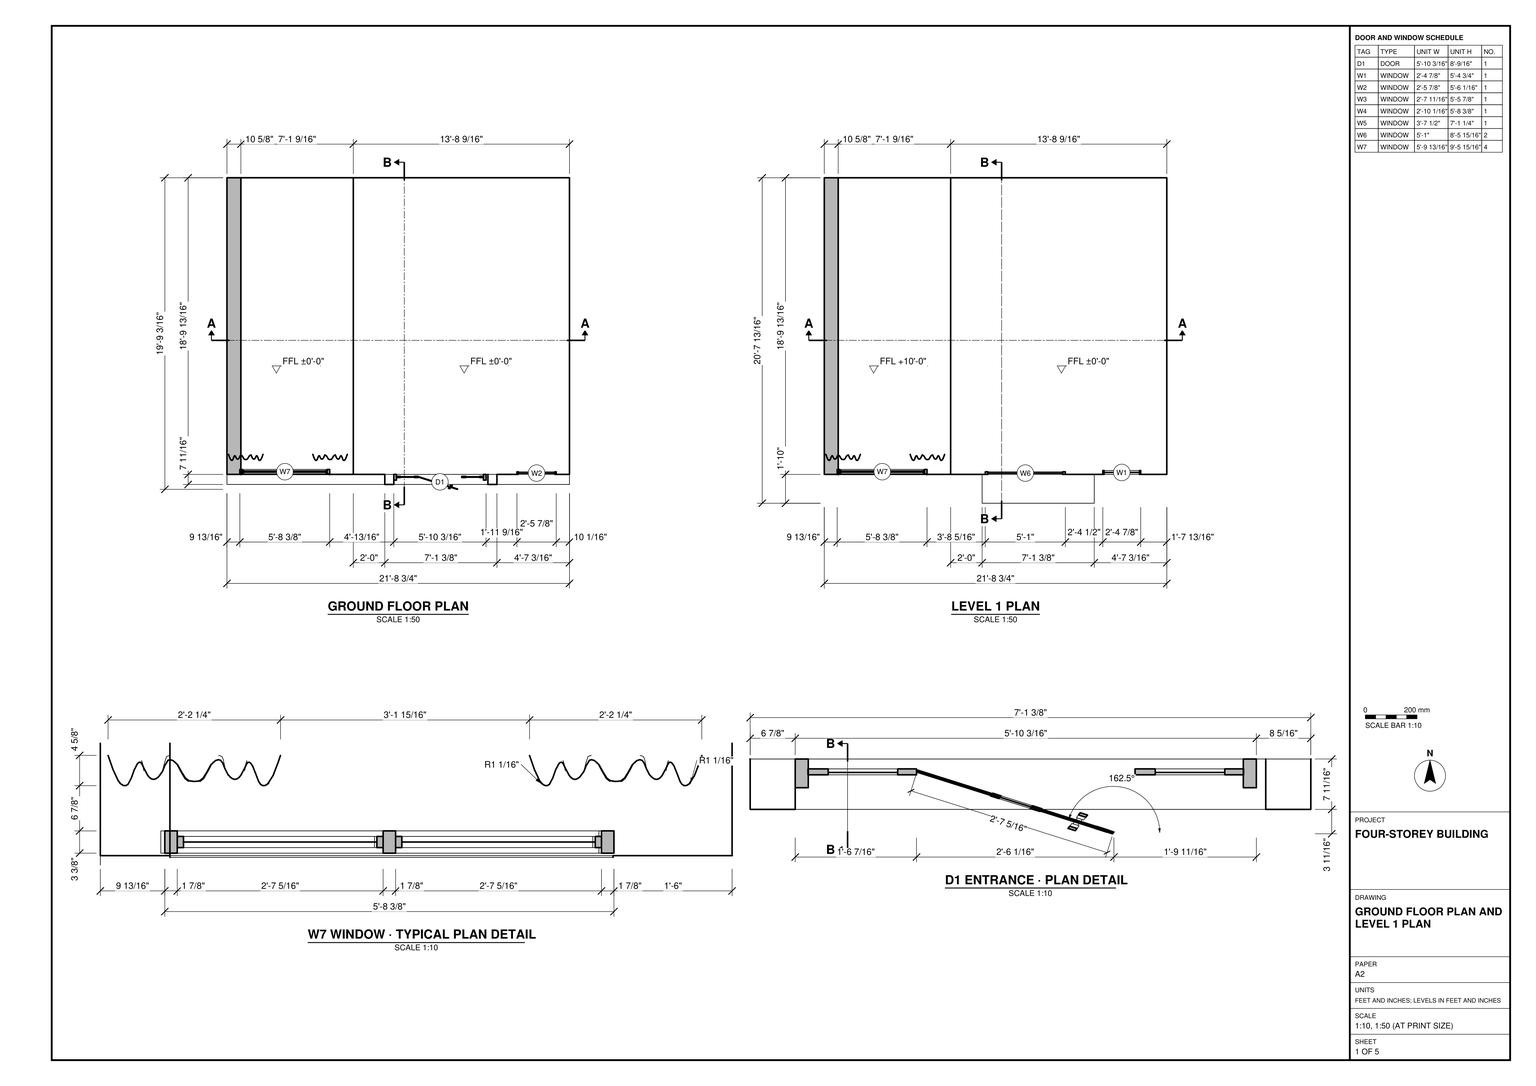
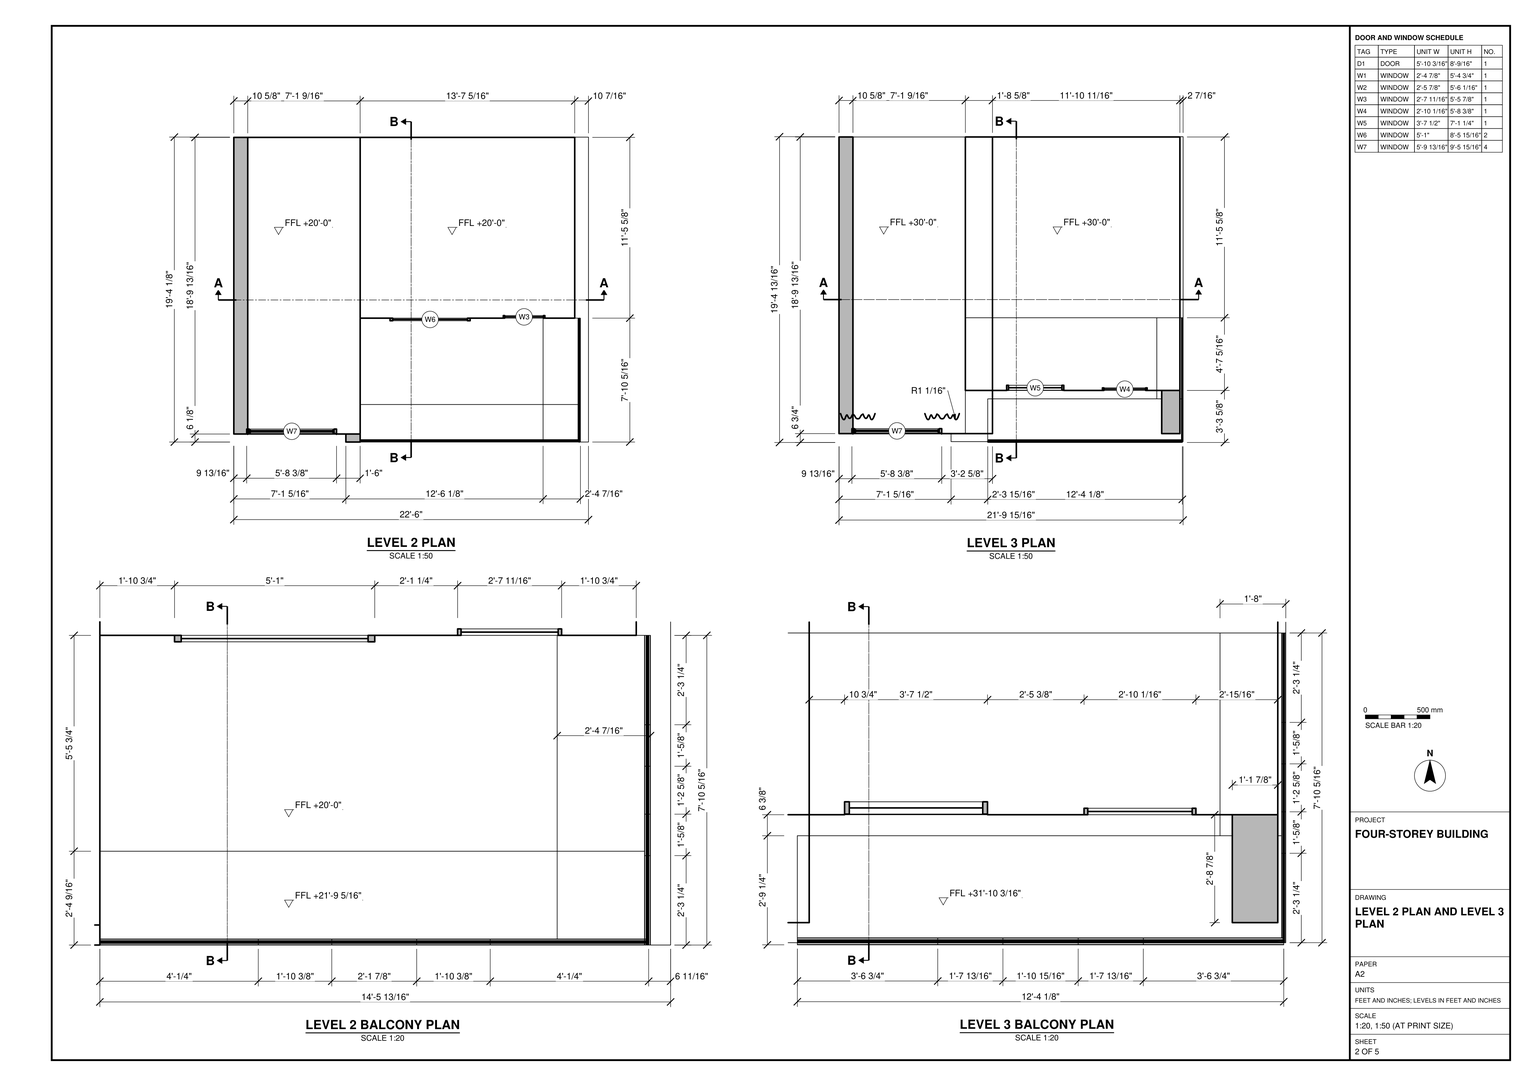
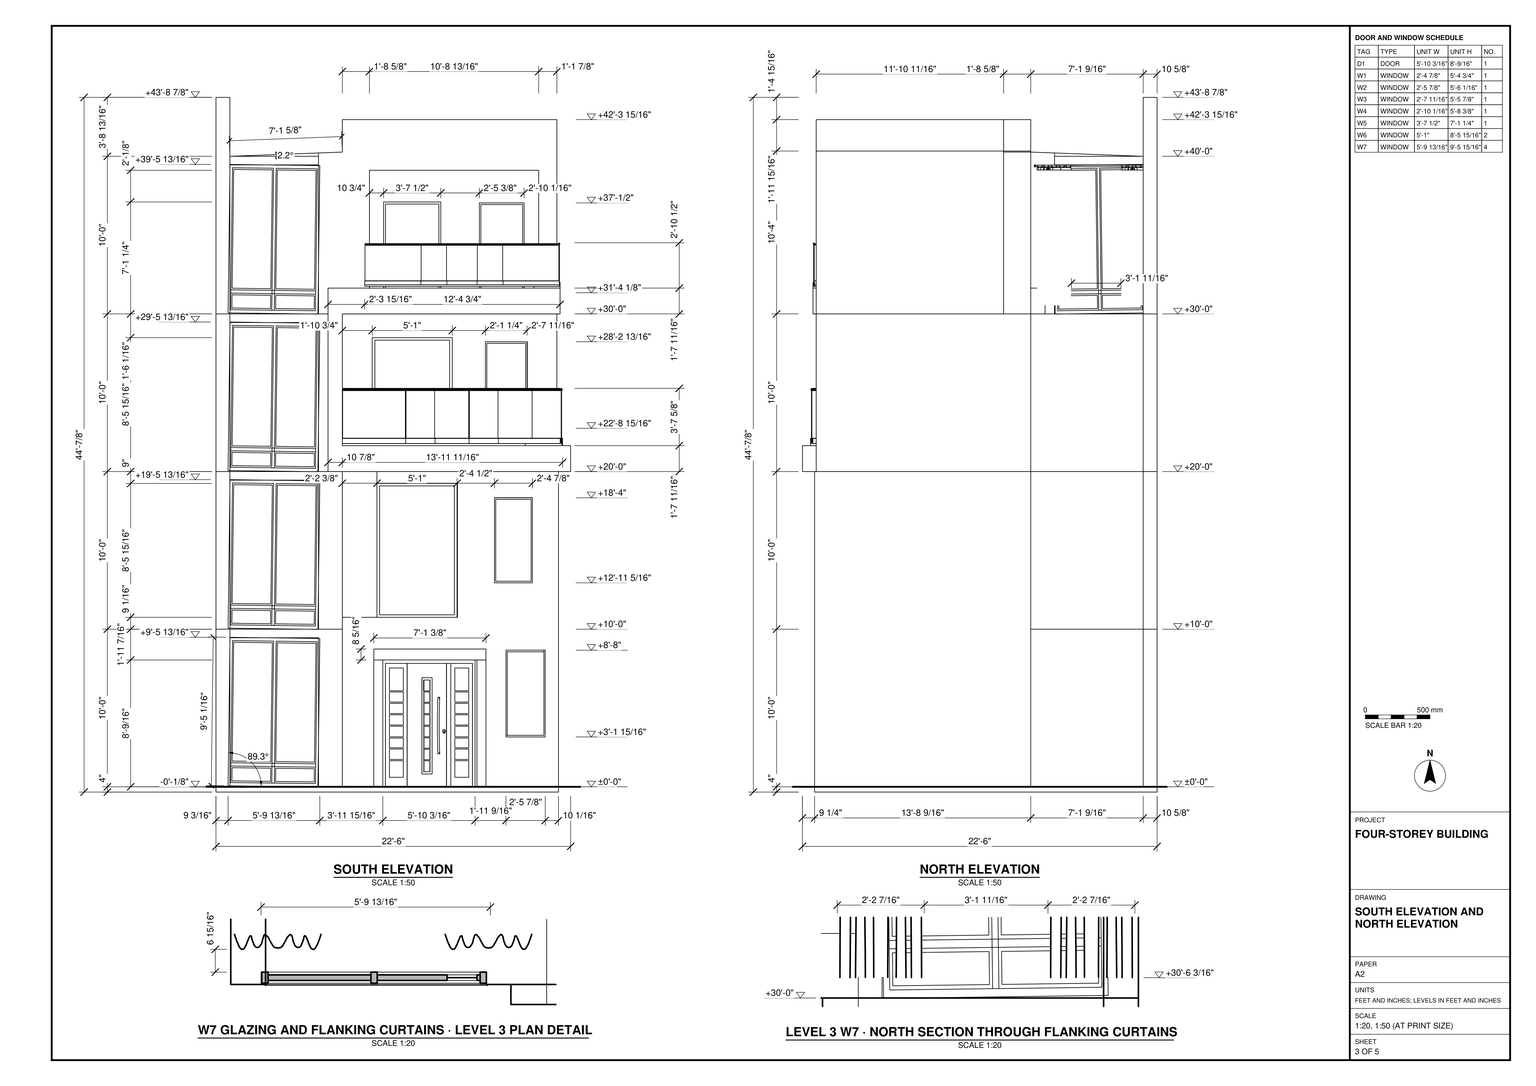
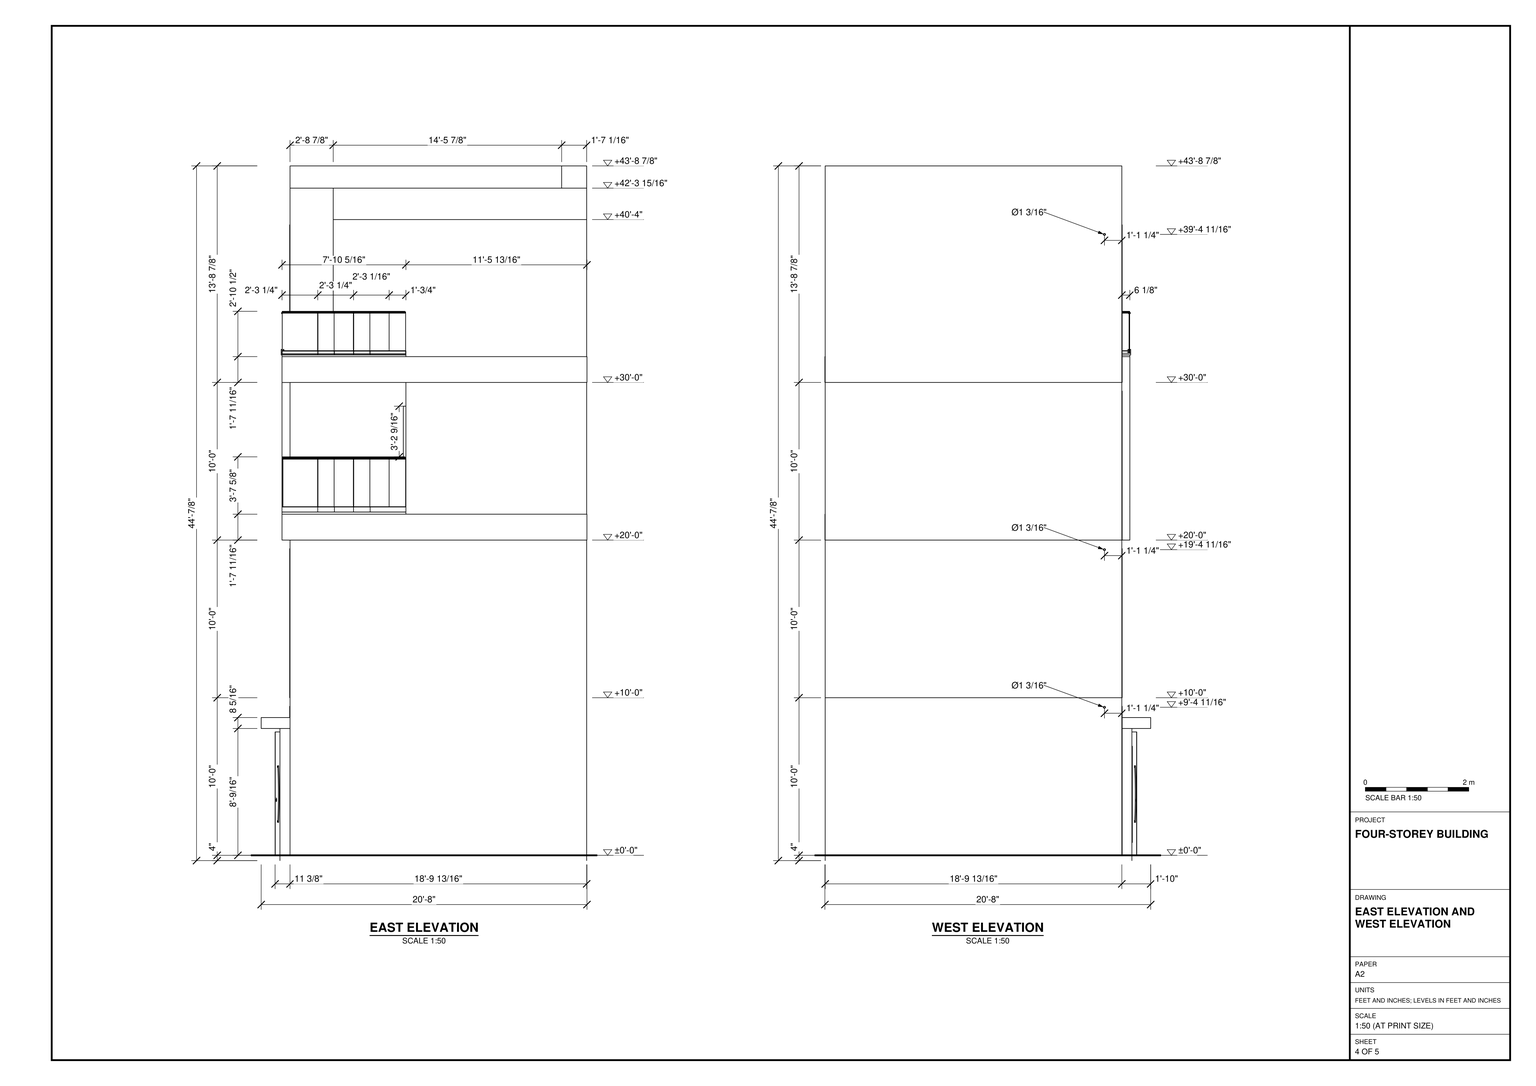
Build the four-storey building in SketchUp from task_files/diagram_01.pdf. Work in feet and inches. The overall extents, including projections, are 22'-6" across the south elevation, 20'-8" from front to back and 44'-7/8" high. Set the ground floor at ±0'-0" and the upper floors at +10'-0", +20'-0" and +30'-0".

Use the plan for each floor to set out its slab edges, wall thicknesses, setbacks and openings. On the south face, stack the tall glazed units in the narrow left bay. Give each unit its centre mullion and low horizontal division. Place the entrance in the wider bay, with glazed side panels and a separate window to the right. Follow the schedule for the window sizes on each floor rather than repeating the whole ground-floor facade.

Model the two upper balconies from their respective enlarged plans, including the slab edges, front glass railings and side returns. Follow the stepped roof outline in elevation, with the shallow slope over the glazed bay and the outer wall rising above it. Any curtains, decor or loose items shown may use suitable library components.

Keep walls, slabs and roof elements separate as groups or components. Keep each furniture or joinery piece separate and use components for repeated parts. Save one SketchUp model as output_files/four_storey_building_with_stacked_glazing_and_balconies.skp.

# SketchUp Ruby script. Lengths in inches.
U = 1.inch
M = Sketchup.active_model
def pt(a) = Geom::Point3d.new(a.map { |v| v * U })
def face(e, loops, mat)
  f = e.add_face(loops[0].map { |a| pt(a) })
  loops[1..].each { |l| e.add_face(l.map { |a| pt(a) }).erase! }
  f.material = f.back_material = mat if mat
  f
end
# faces: each face lists its corners as indices into pts; further lists are holes
def faces(e, pts, list, mat = nil) = list.each { |f| face(e, (f[0].is_a?(Array) ? f : [f]).map { |l| l.map { |i| pts[i] } }, mat) }
# xy, xz, yz: faces in a plane at the given z, y or x. An outline is a flat list of corners, or four numbers for a rectangle; further outlines are holes
def ring(l) = l.size == 4 ? [[l[0], l[1]], [l[2], l[1]], [l[2], l[3]], [l[0], l[3]]] : l.each_slice(2).to_a
def flat(e, list, mat, &to3) = list.each { |f| face(e, (f[0].is_a?(Array) ? f : [f]).map { |l| ring(l).map { |u, v| to3.(u, v) } }, mat) }
def xy(e, z, list, mat = nil) = flat(e, list, mat) { |x, y| [x, y, z] }
def xz(e, y, list, mat = nil) = flat(e, list, mat) { |x, z| [x, y, z] }
def yz(e, x, list, mat = nil) = flat(e, list, mat) { |y, z| [x, y, z] }
def lines(e, pts, list) = list.each { |a, b| e.add_line(pt(pts[a]), pt(pts[b])) }
# prism: a flat outline (further loops are holes) pulled along v
def prism(e, loops, v, mat = nil)
  f = face(e, loops, mat); d = Geom::Vector3d.new(v.map { |x| x * U })
  f.pushpull(f.normal.samedirection?(d) ? d.length : -d.length)
end
def box(e, o, s, mat = nil) = prism(e, [[o, [o[0] + s[0], o[1], o[2]], [o[0] + s[0], o[1] + s[1], o[2]], [o[0], o[1] + s[1], o[2]]]], [0, 0, s[2]], mat)
def at(x, y, z, deg = 0) = Geom::Transformation.translation(pt([x, y, z])) * Geom::Transformation.rotation(ORIGIN, Z_AXIS, deg.degrees)
def axes(o, x, y, z) = Geom::Transformation.new([*x, 0, *y, 0, *z, 0, *pt(o).to_a, 1])
def part(name) = M.definitions.add(name)
# library, detail: a bought-in or finely detailed component or shape, given as its bounding box
def library(name, o, s) = part(name).tap { |d| box(d.entities, o, s) }
def detail(e, o, s) = box(e.add_group.entities, o, s)
def put(e, d, t, mat = nil) = e.add_instance(d, t).tap { |i| i.material = mat if mat }
def group(e, t, mat = nil) = e.add_group.tap { |g| g.transformation = t; g.material = mat if mat }.entities
root = M.entities
M.materials.add("Brick_09_1K").color = [58, 56, 48]
M.materials.add("Brick_09_1K1").color = [234, 224, 191]
M.materials.add("Brick_09_1K2").color = [252, 247, 200]
M.materials.add("Brick_09_1K3").color = [48, 46, 39]
M.materials.add("Brick_09_1K4").color = [244, 233, 199]
M.materials.add("Brick_09_1K5").color = [71, 67, 57]
M.materials.add("D08_Bronzed_Mustard").color = [102, 74, 0]
M.materials.add("Generic").color = [255, 255, 255]
M.materials.add("Tile_Exterior_07_1K1").color = [112, 111, 107]
M.materials.add("[Color A01]").color = [30, 30, 30]
M.materials.add("[Color M07]").color = [58, 58, 58]
M.materials.add("[Metal Corrugated Shiny]2").color = [193, 193, 193]
M.materials.add("[Translucent Glass Blue]").color = [74, 98, 119]
M.materials["[Translucent Glass Blue]"].alpha = 0.8
M.materials.add("[Translucent Glass Gray]").color = [128, 128, 128]
M.materials["[Translucent Glass Gray]"].alpha = 0.5
M.materials.add("[Translucent Glass Gray]3").color = [128, 128, 128]
M.materials["[Translucent Glass Gray]3"].alpha = 0.3
c1 = part("Group\#3")
xy(c1.entities,0,[[0,0,32.48,1.97]])
xy(c1.entities,0.98,[[0.98,0,31.5,0.98],[0.98,0.98,31.5,1.97]])
xy(c1.entities,8.86,[[0.98,0,31.5,0.98],[0.98,0.98,31.5,1.97]])
xy(c1.entities,9.84,[[0,0,32.48,1.97]])
xz(c1.entities,0,[[[0,0,32.48,9.84],[0.98,0.98,31.5,8.86]]])
xz(c1.entities,0.98,[[0.98,0.98,31.5,8.86]],"[Translucent Glass Gray]")
xz(c1.entities,1.97,[[[0,0,32.48,9.84],[0.98,0.98,31.5,8.86]]])
yz(c1.entities,0,[[0,0,1.97,9.84]])
yz(c1.entities,0.98,[[0,0.98,0.98,8.86],[0.98,0.98,1.97,8.86]])
yz(c1.entities,31.5,[[0,0.98,0.98,8.86],[0.98,0.98,1.97,8.86]])
yz(c1.entities,32.48,[[0,0,1.97,9.84]])
c2 = part("Group\#4")
xy(c2.entities,0,[[0,0,32.48,1.97]])
xy(c2.entities,0.98,[[0.98,0,31.5,0.98],[0.98,0.98,31.5,1.97]])
xy(c2.entities,71.85,[[0.98,0,31.5,0.98],[0.98,0.98,31.5,1.97]])
xy(c2.entities,72.83,[[0,0,32.48,1.97]])
xz(c2.entities,0,[[[0,0,32.48,72.83],[0.98,0.98,31.5,71.85]]])
xz(c2.entities,0.98,[[0.98,0.98,31.5,71.85]],"[Translucent Glass Gray]")
xz(c2.entities,1.97,[[[0,0,32.48,72.83],[0.98,0.98,31.5,71.85]]])
yz(c2.entities,0,[[0,0,1.97,72.83]])
yz(c2.entities,0.98,[[0,0.98,0.98,71.85],[0.98,0.98,1.97,71.85]])
yz(c2.entities,31.5,[[0,0.98,0.98,71.85],[0.98,0.98,1.97,71.85]])
yz(c2.entities,32.48,[[0,0,1.97,72.83]])
c3 = part("FIXED GLASS WINDOW WITH TRANSOM")
g1 = group(c3.entities,at(0,0,0))
xy(g1,0,[[0,0,70.86,3.9375]])
xy(g1,1.97,[[1.97,0,34.45,0.98],[36.42,0,68.9,3.9375],[1.97,2.95,34.45,3.9375]])
xy(g1,86.61,[[1.97,0,34.45,3.9375],[34.45,0,36.42,3.9375],[36.42,0,68.9,3.9375]])
xy(g1,88.58,[[0,0,70.86,3.9375]])
xz(g1,0,[[[0,0,70.86,88.58],[1.97,1.97,34.45,86.61],[36.42,1.97,68.9,86.61]]])
xz(g1,3.9375,[[[0,0,70.86,88.58],[1.97,1.97,34.45,86.61],[36.42,1.97,68.9,86.61]]])
yz(g1,0,[[0,0,3.9375,88.58]])
yz(g1,1.97,[[0,1.97,3.9375,74.8],[0,76.77,3.9375,86.61]])
yz(g1,34.45,[[0,1.97,3.9375,86.61]])
yz(g1,36.42,[[0,1.97,3.9375,86.61]])
yz(g1,68.9,[[0,1.97,3.9375,86.61]])
yz(g1,70.86,[[0,0,3.9375,88.58]])
g2 = group(g1,at(1.97,0,74.8))
box(g2,[0,0,0],[66.93,3.9375,1.97])
put(g1,c1,at(1.97,0.98,76.77))
put(g1,c1,at(36.42,0.98,76.77))
put(g1,c2,at(1.97,0.98,1.97))
put(g1,c2,at(36.42,0.98,1.97))
c4 = library("fronceur aubin blanc",[-47.99,-0.29,1.66],[95.37,4.84,114.09])
c5 = part("Laterais")
xy(c5.entities,0,[[0,0,151.17,12.99]],"D08_Bronzed_Mustard")
xy(c5.entities,50.18,[[28.125,0,124.98,5.12],[28.125,5.12,124.98,12.99]],"D08_Bronzed_Mustard")
xy(c5.entities,137.63,[[28.125,0,124.98,5.12],[28.125,5.12,124.98,12.99]],"D08_Bronzed_Mustard")
xy(c5.entities,144.15,[[28.125,0,124.98,5.12],[28.125,5.12,124.98,12.99]],"D08_Bronzed_Mustard")
xy(c5.entities,199.05,[[28.125,0,124.98,5.12],[28.125,5.12,124.98,12.99]],"D08_Bronzed_Mustard")
xy(c5.entities,205.57,[[28.125,0,124.98,5.12],[28.125,5.12,124.98,12.99]],"D08_Bronzed_Mustard")
xy(c5.entities,256.92,[[28.125,0,124.98,5.12],[28.125,5.12,124.98,12.99]],"D08_Bronzed_Mustard")
xy(c5.entities,263.44,[[28.125,0,124.98,5.12],[28.125,5.12,124.98,12.99]],"D08_Bronzed_Mustard")
xy(c5.entities,319.125,[[28.125,0,124.98,5.12],[28.125,5.12,124.98,12.99]],"D08_Bronzed_Mustard")
xy(c5.entities,325.64,[[28.125,0,124.98,5.12],[28.125,5.12,124.98,12.99]],"D08_Bronzed_Mustard")
xy(c5.entities,379.76,[[28.125,0,124.98,5.12],[28.125,5.12,124.98,12.99]],"D08_Bronzed_Mustard")
xy(c5.entities,386.27,[[28.125,0,124.98,5.12],[28.125,5.12,124.98,12.99]],"D08_Bronzed_Mustard")
xy(c5.entities,439.99,[[28.125,0,124.98,5.12],[28.125,5.12,124.98,12.99]],"D08_Bronzed_Mustard")
xy(c5.entities,446.51,[[28.125,0,124.98,5.12],[28.125,5.12,124.98,12.99]],"D08_Bronzed_Mustard")
xy(c5.entities,499.82,[[28.125,0,124.98,5.12],[28.125,5.12,124.98,12.99]],"D08_Bronzed_Mustard")
xy(c5.entities,506.17,[[28.125,0,124.98,5.12],[28.125,5.12,124.98,12.99]],"D08_Bronzed_Mustard")
xy(c5.entities,626.16,[[28.125,0,124.98,5.12],[28.125,5.12,124.98,12.99]],"D08_Bronzed_Mustard")
xy(c5.entities,650.39,[[0,0,151.17,12.99]],"D08_Bronzed_Mustard")
xz(c5.entities,0,[[[0,0,151.17,650.39],[28.125,506.17,124.98,626.16],[28.125,50.18,124.98,137.63],[28.125,263.44,124.98,319.125],[28.125,144.15,124.98,199.05],[28.125,325.64,124.98,379.76],[28.125,386.27,124.98,439.99],[28.125,446.51,124.98,499.82],[28.125,205.57,124.98,256.92]]],"D08_Bronzed_Mustard")
xz(c5.entities,5.12,[[28.125,50.18,124.98,137.63],[28.125,144.15,124.98,199.05],[28.125,205.57,124.98,256.92],[28.125,263.44,124.98,319.125],[28.125,325.64,124.98,379.76],
  [28.125,386.27,124.98,439.99],[28.125,446.51,124.98,499.82],[28.125,506.17,124.98,626.16]],"[Translucent Glass Blue]")
xz(c5.entities,12.99,[[[0,0,151.17,650.39],[28.125,506.17,124.98,626.16],[28.125,50.18,124.98,137.63],[28.125,263.44,124.98,319.125],[28.125,144.15,124.98,199.05],[28.125,325.64,124.98,379.76],[28.125,386.27,124.98,439.99],[28.125,446.51,124.98,499.82],[28.125,205.57,124.98,256.92]]],"D08_Bronzed_Mustard")
yz(c5.entities,0,[[0,0,12.99,650.39]],"D08_Bronzed_Mustard")
yz(c5.entities,28.125,[[0,50.18,5.12,137.63],[5.12,50.18,12.99,137.63],[0,144.15,5.12,199.05],[5.12,144.15,12.99,199.05],[0,205.57,5.12,256.92],
  [5.12,205.57,12.99,256.92],[0,263.44,5.12,319.125],[5.12,263.44,12.99,319.125],[0,325.64,5.12,379.76],[5.12,325.64,12.99,379.76],
  [0,386.27,5.12,439.99],[5.12,386.27,12.99,439.99],[0,446.51,5.12,499.82],[5.12,446.51,12.99,499.82],[0,506.17,5.12,626.16],
  [5.12,506.17,12.99,626.16]],"D08_Bronzed_Mustard")
yz(c5.entities,124.98,[[0,50.18,5.12,137.63],[5.12,50.18,12.99,137.63],[0,144.15,5.12,199.05],[5.12,144.15,12.99,199.05],[0,205.57,5.12,256.92],
  [5.12,205.57,12.99,256.92],[0,263.44,5.12,319.125],[5.12,263.44,12.99,319.125],[0,325.64,5.12,379.76],[5.12,325.64,12.99,379.76],
  [0,386.27,5.12,439.99],[5.12,386.27,12.99,439.99],[0,446.51,5.12,499.82],[5.12,446.51,12.99,499.82],[0,506.17,5.12,626.16],
  [5.12,506.17,12.99,626.16]],"D08_Bronzed_Mustard")
yz(c5.entities,151.17,[[0,0,12.99,650.39]],"D08_Bronzed_Mustard")
c6 = part("Agrupar\#1")
xy(c6.entities,0,[[12.72,5.49,9.61,6.17,6.78,7.65,4.43,9.8,2.72,12.49,1.76,15.52,1.625,18.71,2.31,21.82,3.79,24.64,5.9375,26.99,8.625,28.7,11.66,29.66,14.85,29.8,17.96,29.11,20.78,27.64,23.13,25.49,24.84,22.8,25.8,19.76,25.94,16.58,25.25,13.47,23.78,10.64,21.63,8.29,18.94,6.58,15.9,5.625],[765.48,5.49,762.37,6.17,759.54,7.65,757.19,9.8,755.48,12.49,754.52,15.52,754.38,18.71,755.07,21.82,756.54,24.64,758.69,26.99,761.38,28.7,764.42,29.66,767.6,29.8,770.71,29.11,773.54,27.64,775.89,25.49,777.6,22.8,778.56,19.76,778.7,16.58,778.01,13.47,776.54,10.64,774.38,8.29,771.7,6.58,768.66,5.625]],"[Metal Corrugated Shiny]2")
xy(c6.entities,39.37,[[[0,0,27.28,36.52],[12.72,5.49,15.9,5.625,18.94,6.58,21.63,8.29,23.78,10.64,25.25,13.47,25.94,16.58,25.8,19.76,24.84,22.8,23.13,25.49,20.78,27.64,17.96,29.11,14.85,29.8,11.66,29.66,8.625,28.7,5.9375,26.99,3.79,24.64,2.31,21.82,1.625,18.71,1.76,15.52,2.72,12.49,4.43,9.8,6.78,7.65,9.61,6.17]],[[753.42,0,780.71,36.52],[765.48,5.49,768.66,5.625,771.7,6.58,774.38,8.29,776.54,10.64,778.01,13.47,778.7,16.58,778.56,19.76,777.6,22.8,775.89,25.49,773.54,27.64,770.71,29.11,767.6,29.8,764.42,29.66,761.38,28.7,758.69,26.99,756.54,24.64,755.07,21.82,754.38,18.71,754.52,15.52,755.48,12.49,757.19,9.8,759.54,7.65,762.37,6.17]]],"[Metal Corrugated Shiny]2")
xz(c6.entities,0,[[0,39.37,27.28,39.37,68.875,46.96,132.75,56.47,196.91,63.88,261.28,69.18,325.78,72.36,390.35,73.42,454.93,72.36,519.43,69.18,583.8,63.88,647.96,56.47,711.83,46.96,753.42,39.37,780.71,39.37,780.71,62.125,716.29,73.89,651.53,83.53,586.48,91.04,521.22,96.41,455.82,99.63,390.35,100.71,324.88,99.63,259.48,96.41,194.23,91.04,129.18,83.53,64.41,73.89,0,62.125]],"[Metal Corrugated Shiny]2")
xz(c6.entities,36.52,[[0,39.37,0,62.125,64.41,73.89,129.18,83.53,194.23,91.04,259.48,96.41,324.88,99.63,390.35,100.71,455.82,99.63,521.22,96.41,586.48,91.04,651.53,83.53,716.29,73.89,780.71,62.125,780.71,39.37,753.42,39.37,711.83,46.96,647.96,56.47,583.8,63.88,519.43,69.18,454.93,72.36,390.35,73.42,325.78,72.36,261.28,69.18,196.91,63.88,132.75,56.47,68.875,46.96,27.28,39.37]],"[Metal Corrugated Shiny]2")
yz(c6.entities,0,[[0,39.37,36.52,62.125]],"[Metal Corrugated Shiny]2")
yz(c6.entities,780.71,[[0,39.37,36.52,62.125]],"[Metal Corrugated Shiny]2")
p = [[12.72,5.49,39.37],[9.61,6.17,39.37],[9.61,6.17,0],[12.72,5.49,0],[15.9,5.625,39.37],[15.9,5.625,0],
  [765.48,5.49,39.37],[762.37,6.17,39.37],[762.37,6.17,0],[765.48,5.49,0],[768.66,5.625,39.37],[768.66,5.625,0],
  [18.94,6.58,39.37],[18.94,6.58,0],[771.7,6.58,39.37],[771.7,6.58,0],[6.78,7.65,39.37],[6.78,7.65,0],
  [759.54,7.65,39.37],[759.54,7.65,0],[21.63,8.29,39.37],[21.63,8.29,0],[774.38,8.29,39.37],[774.38,8.29,0],
  [4.43,9.8,39.37],[4.43,9.8,0],[757.19,9.8,39.37],[757.19,9.8,0],[23.78,10.64,39.37],[23.78,10.64,0],
  [776.54,10.64,39.37],[776.54,10.64,0],[2.72,12.49,39.37],[2.72,12.49,0],[755.48,12.49,39.37],[755.48,12.49,0],
  [25.25,13.47,39.37],[25.25,13.47,0],[778.01,13.47,39.37],[778.01,13.47,0],[1.76,15.52,39.37],[1.76,15.52,0],
  [754.52,15.52,39.37],[754.52,15.52,0],[25.94,16.58,39.37],[25.94,16.58,0],[778.7,16.58,39.37],[778.7,16.58,0],
  [1.625,18.71,39.37],[1.625,18.71,0],[754.38,18.71,39.37],[754.38,18.71,0],[25.8,19.76,39.37],[25.8,19.76,0],
  [778.56,19.76,39.37],[778.56,19.76,0],[2.31,21.82,39.37],[2.31,21.82,0],[755.07,21.82,39.37],[755.07,21.82,0],
  [24.84,22.8,39.37],[24.84,22.8,0],[777.6,22.8,39.37],[777.6,22.8,0],[3.79,24.64,39.37],[3.79,24.64,0],
  [756.54,24.64,39.37],[756.54,24.64,0],[23.13,25.49,39.37],[23.13,25.49,0],[775.89,25.49,39.37],[775.89,25.49,0],
  [5.9375,26.99,39.37],[5.9375,26.99,0],[758.69,26.99,39.37],[758.69,26.99,0],[20.78,27.64,39.37],[20.78,27.64,0],
  [773.54,27.64,39.37],[773.54,27.64,0],[8.625,28.7,39.37],[8.625,28.7,0],[761.38,28.7,39.37],[761.38,28.7,0],
  [17.96,29.11,39.37],[17.96,29.11,0],[770.71,29.11,39.37],[770.71,29.11,0],[11.66,29.66,39.37],[11.66,29.66,0],
  [764.42,29.66,39.37],[764.42,29.66,0],[14.85,29.8,39.37],[14.85,29.8,0],[767.6,29.8,39.37],[767.6,29.8,0],
  [68.875,0,46.96],[27.28,0,39.37],[27.28,36.52,39.37],[68.875,36.52,46.96],[753.42,0,39.37],[711.83,0,46.96],
  [711.83,36.52,46.96],[753.42,36.52,39.37],[132.75,0,56.47],[132.75,36.52,56.47],[647.96,0,56.47],[647.96,36.52,56.47],
  [196.91,0,63.88],[196.91,36.52,63.88],[583.8,0,63.88],[583.8,36.52,63.88],[0,0,62.125],[64.41,0,73.89],
  [64.41,36.52,73.89],[0,36.52,62.125],[716.29,0,73.89],[780.71,0,62.125],[780.71,36.52,62.125],[716.29,36.52,73.89],
  [261.28,0,69.18],[261.28,36.52,69.18],[519.43,0,69.18],[519.43,36.52,69.18],[325.78,0,72.36],[325.78,36.52,72.36],
  [454.93,0,72.36],[454.93,36.52,72.36],[390.35,0,73.42],[390.35,36.52,73.42],[129.18,0,83.53],[129.18,36.52,83.53],
  [651.53,0,83.53],[651.53,36.52,83.53],[194.23,0,91.04],[194.23,36.52,91.04],[586.48,0,91.04],[586.48,36.52,91.04],
  [259.48,0,96.41],[259.48,36.52,96.41],[521.22,0,96.41],[521.22,36.52,96.41],[324.88,0,99.63],[324.88,36.52,99.63],
  [455.82,0,99.63],[455.82,36.52,99.63],[390.35,0,100.71],[390.35,36.52,100.71]]
faces(c6.entities,p,[[0,1,2,3],[4,0,3,5],[6,7,8,9],[10,6,9,11],[12,4,5,13],[14,10,11,15],[1,16,17,2],[7,18,19,8],
  [20,12,13,21],[22,14,15,23],[16,24,25,17],[18,26,27,19],[28,20,21,29],[30,22,23,31],[24,32,33,25],[26,34,35,27],
  [36,28,29,37],[38,30,31,39],[32,40,41,33],[34,42,43,35],[44,36,37,45],[46,38,39,47],[40,48,49,41],[42,50,51,43],
  [52,44,45,53],[54,46,47,55],[48,56,57,49],[50,58,59,51],[60,52,53,61],[62,54,55,63],[56,64,65,57],[58,66,67,59],
  [68,60,61,69],[70,62,63,71],[64,72,73,65],[66,74,75,67],[76,68,69,77],[78,70,71,79],[72,80,81,73],[74,82,83,75],
  [84,76,77,85],[86,78,79,87],[80,88,89,81],[82,90,91,83],[92,84,85,93],[94,86,87,95],[88,92,93,89],[90,94,95,91],
  [96,97,98,99],[100,101,102,103],[104,96,99,105],[101,106,107,102],[108,104,105,109],[106,110,111,107],[112,113,114,115],[116,117,118,119],
  [120,108,109,121],[110,122,123,111],[124,120,121,125],[122,126,127,123],[128,124,125,129],[126,128,129,127],[113,130,131,114],[132,116,119,133],
  [130,134,135,131],[136,132,133,137],[134,138,139,135],[140,136,137,141],[138,142,143,139],[144,140,141,145],[142,146,147,143],[146,144,145,147]],"[Metal Corrugated Shiny]2")
c7 = part("Puxador")
put(c7.entities,c6,at(-239.95,414.09,8.74))
c8 = part("Pt 03")
xy(c8.entities,0,[[0,17.04,314.27,19.21],[0,19.21,314.27,21.375]],"Generic")
xy(c8.entities,67.57,[[119.26,15.86,198.39,17.04],[119.26,21.375,198.39,22.56]],"Generic")
xy(c8.entities,79.4,[[132.64,15.86,183.04,19.21],[132.64,19.21,183.04,22.56]],"Generic")
xy(c8.entities,137.44,[[132.64,15.86,183.04,19.21],[132.64,19.21,183.04,22.56]],"Generic")
xy(c8.entities,142.82,[[132.64,15.86,183.04,19.21],[132.64,19.21,183.04,22.56]],"Generic")
xy(c8.entities,197.68,[[132.64,15.86,183.04,19.21],[132.64,19.21,183.04,22.56]],"Generic")
xy(c8.entities,203.05,[[132.64,15.86,183.04,19.21],[132.64,19.21,183.04,22.56]],"Generic")
xy(c8.entities,258.31,[[132.64,15.86,183.04,19.21],[132.64,19.21,183.04,22.56]],"Generic")
xy(c8.entities,263.68,[[132.64,15.86,183.04,19.21],[132.64,19.21,183.04,22.56]],"Generic")
xy(c8.entities,285.78,[[294.1,15.82,298.33,17.04],[294.1,21.375,298.33,22.6]],"Generic")
xy(c8.entities,319.33,[[132.64,15.86,183.04,19.21],[132.64,19.21,183.04,22.56]],"Generic")
xy(c8.entities,324.71,[[132.64,15.86,183.04,19.21],[132.64,19.21,183.04,22.56]],"Generic")
xy(c8.entities,379.96,[[132.64,15.86,183.04,19.21],[132.64,19.21,183.04,22.56]],"Generic")
xy(c8.entities,385.34,[[132.64,15.86,183.04,19.21],[132.64,19.21,183.04,22.56]],"Generic")
xy(c8.entities,440.2,[[132.64,15.86,183.04,19.21],[132.64,19.21,183.04,22.56]],"Generic")
xy(c8.entities,445.57,[[132.64,15.86,183.04,19.21],[132.64,19.21,183.04,22.56]],"Generic")
xy(c8.entities,500.04,[[132.64,15.86,183.04,19.21],[132.64,19.21,183.04,22.56]],"Generic")
xy(c8.entities,505.41,[[132.53,15.86,132.64,19.21],[132.64,15.86,182.93,19.21],[132.53,19.21,182.93,22.56]],"Generic")
xy(c8.entities,562.86,[[132.64,15.86,182.93,19.21],[182.93,15.86,183.04,19.21],[132.64,19.21,183.04,22.56]],"Generic")
xy(c8.entities,575.05,[[119.26,15.86,198.39,17.04],[119.26,21.375,198.39,22.56]],"Generic")
xy(c8.entities,650.39,[[0,17.04,314.27,19.21],[0,19.21,314.27,21.375]],"Generic")
xz(c8.entities,15.82,[[[294.8,282.65,297.37,282.74,299.84,283.48,302.02,284.84,303.79,286.72,305,288.99,305.59,291.5,305.5,294.07,304.76,296.54,303.4,298.73,301.52,300.49,299.25,301.7,296.74,302.29,294.17,302.21,291.7,301.46,289.51,300.1,287.75,298.22,286.54,295.95,285.95,293.44,286.03,290.87,286.78,288.41,288.14,286.22,290.02,284.46,292.29,283.24],[294.1,285.78,295.2,290.51,294.44,290.84,293.79,291.35,293.3,292.02,292.99,292.79,292.9,293.61,293.02,294.43,293.35,295.1875,293.86,295.84,294.52,296.33,295.29,296.64,296.12,296.73,296.9375,296.61,297.7,296.28,298.34,295.77,298.84,295.1,299.14,294.33,299.24,293.51,299.12,292.69,298.79,291.93,298.28,291.28,297.61,290.79,296.84,290.49,298.33,285.78]]],"Generic")
xz(c8.entities,15.86,[[[119.26,67.57,198.39,575.05],[132.64,79.4,183.04,137.44],[132.53,505.41,132.64,562.86,183.04,562.86,182.93,505.41],[132.64,263.68,183.04,319.33],[132.64,324.71,183.04,379.96],[132.64,203.05,183.04,258.31],[132.64,385.34,183.04,440.2],[132.64,142.82,183.04,197.68],[132.64,445.57,183.04,500.04]],[132.53,505.41,132.64,505.41,132.64,562.86],[182.93,505.41,183.04,562.86,182.93,562.86]],"Generic")
xz(c8.entities,17.04,[[[0,0,314.27,650.39],[119.26,67.57,198.39,575.05],[294.8,282.65,292.29,283.24,290.02,284.46,288.14,286.22,286.78,288.41,286.03,290.87,285.95,293.44,286.54,295.95,287.75,298.22,289.51,300.1,291.7,301.46,294.17,302.21,296.74,302.29,299.25,301.7,301.52,300.49,303.4,298.73,304.76,296.54,305.5,294.07,305.59,291.5,305,288.99,303.79,286.72,302.02,284.84,299.84,283.48,297.37,282.74]],[294.1,285.78,298.33,285.78,296.84,290.49,297.61,290.79,298.28,291.28,298.79,291.93,299.12,292.69,299.24,293.51,299.14,294.33,298.84,295.1,298.34,295.77,297.7,296.28,296.9375,296.61,296.12,296.73,295.29,296.64,294.52,296.33,293.86,295.84,293.35,295.1875,293.02,294.43,292.9,293.61,292.99,292.79,293.3,292.02,293.79,291.35,294.44,290.84,295.2,290.51]],"Generic")
xz(c8.entities,19.21,[[[0,0,314.27,650.39],[132.64,79.4,183.04,137.44],[132.53,505.41,182.93,505.41,183.04,562.86,132.64,562.86],[132.64,263.68,183.04,319.33],[132.64,324.71,183.04,379.96],[132.64,203.05,183.04,258.31],[132.64,385.34,183.04,440.2],[132.64,142.82,183.04,197.68],[132.64,445.57,183.04,500.04]],[132.64,79.4,183.04,137.44],[132.64,142.82,183.04,197.68],[132.64,203.05,183.04,258.31],[132.64,263.68,183.04,319.33],
  [132.64,324.71,183.04,379.96],[132.64,385.34,183.04,440.2],[132.64,445.57,183.04,500.04],[132.64,505.41,182.93,562.86]],"Generic")
xz(c8.entities,21.375,[[[0,0,314.27,650.39],[119.26,67.57,198.39,575.05],[294.8,282.65,297.37,282.74,299.84,283.48,302.02,284.84,303.79,286.72,305,288.99,305.59,291.5,305.5,294.07,304.76,296.54,303.4,298.73,301.52,300.49,299.25,301.7,296.74,302.29,294.17,302.21,291.7,301.46,289.51,300.1,287.75,298.22,286.54,295.95,285.95,293.44,286.03,290.87,286.78,288.41,288.14,286.22,290.02,284.46,292.29,283.24]],[294.1,285.78,295.2,290.51,294.44,290.84,293.79,291.35,293.3,292.02,292.99,292.79,292.9,293.61,293.02,294.43,293.35,295.1875,293.86,295.84,294.52,296.33,295.29,296.64,296.12,296.73,296.9375,296.61,297.7,296.28,298.34,295.77,298.84,295.1,299.14,294.33,299.24,293.51,299.12,292.69,298.79,291.93,298.28,291.28,297.61,290.79,296.84,290.49,298.33,285.78]],"Generic")
xz(c8.entities,22.56,[[[119.26,67.57,198.39,575.05],[132.64,79.4,183.04,137.44],[132.53,505.41,182.93,505.41,183.04,562.86,132.64,562.86],[132.64,263.68,183.04,319.33],[132.64,324.71,183.04,379.96],[132.64,203.05,183.04,258.31],[132.64,385.34,183.04,440.2],[132.64,142.82,183.04,197.68],[132.64,445.57,183.04,500.04]]],"Generic")
xz(c8.entities,22.6,[[[294.8,282.65,292.29,283.24,290.02,284.46,288.14,286.22,286.78,288.41,286.03,290.87,285.95,293.44,286.54,295.95,287.75,298.22,289.51,300.1,291.7,301.46,294.17,302.21,296.74,302.29,299.25,301.7,301.52,300.49,303.4,298.73,304.76,296.54,305.5,294.07,305.59,291.5,305,288.99,303.79,286.72,302.02,284.84,299.84,283.48,297.37,282.74],[294.1,285.78,298.33,285.78,296.84,290.49,297.61,290.79,298.28,291.28,298.79,291.93,299.12,292.69,299.24,293.51,299.14,294.33,298.84,295.1,298.34,295.77,297.7,296.28,296.9375,296.61,296.12,296.73,295.29,296.64,294.52,296.33,293.86,295.84,293.35,295.1875,293.02,294.43,292.9,293.61,292.99,292.79,293.3,292.02,293.79,291.35,294.44,290.84,295.2,290.51]]],"Generic")
yz(c8.entities,0,[[17.04,0,19.21,650.39],[19.21,0,21.375,650.39]],"Generic")
yz(c8.entities,119.26,[[15.86,67.57,17.04,575.05],[21.375,67.57,22.56,575.05]],"Generic")
yz(c8.entities,132.64,[[15.86,79.4,19.21,137.44],[19.21,79.4,22.56,137.44],[15.86,142.82,19.21,197.68],[19.21,142.82,22.56,197.68],[15.86,203.05,19.21,258.31],
  [19.21,203.05,22.56,258.31],[15.86,263.68,19.21,319.33],[19.21,263.68,22.56,319.33],[15.86,324.71,19.21,379.96],[19.21,324.71,22.56,379.96],
  [15.86,385.34,19.21,440.2],[19.21,385.34,22.56,440.2],[15.86,445.57,19.21,500.04],[19.21,445.57,22.56,500.04],[15.86,505.41,19.21,562.86]],"Generic")
yz(c8.entities,182.93,[[15.86,505.41,19.21,562.86]],"Generic")
yz(c8.entities,183.04,[[15.86,79.4,19.21,137.44],[19.21,79.4,22.56,137.44],[15.86,142.82,19.21,197.68],[19.21,142.82,22.56,197.68],[15.86,203.05,19.21,258.31],
  [19.21,203.05,22.56,258.31],[15.86,263.68,19.21,319.33],[19.21,263.68,22.56,319.33],[15.86,324.71,19.21,379.96],[19.21,324.71,22.56,379.96],
  [15.86,385.34,19.21,440.2],[19.21,385.34,22.56,440.2],[15.86,445.57,19.21,500.04],[19.21,445.57,22.56,500.04]],"Generic")
yz(c8.entities,198.39,[[15.86,67.57,17.04,575.05],[21.375,67.57,22.56,575.05]],"Generic")
yz(c8.entities,314.27,[[17.04,0,19.21,650.39],[19.21,0,21.375,650.39]],"Generic")
p = [[292.29,17.04,283.24],[294.8,17.04,282.65],[294.8,15.82,282.65],[292.29,15.82,283.24],[297.37,17.04,282.74],[297.37,15.82,282.74],
  [299.84,17.04,283.48],[299.84,15.82,283.48],[294.8,21.375,282.65],[292.29,21.375,283.24],[292.29,22.6,283.24],[294.8,22.6,282.65],
  [297.37,21.375,282.74],[297.37,22.6,282.74],[299.84,21.375,283.48],[299.84,22.6,283.48],[290.02,17.04,284.46],[290.02,15.82,284.46],
  [290.02,21.375,284.46],[290.02,22.6,284.46],[302.02,17.04,284.84],[302.02,15.82,284.84],[302.02,21.375,284.84],[302.02,22.6,284.84],
  [288.14,17.04,286.22],[288.14,15.82,286.22],[288.14,21.375,286.22],[288.14,22.6,286.22],[303.79,17.04,286.72],[303.79,15.82,286.72],
  [303.79,21.375,286.72],[303.79,22.6,286.72],[295.2,15.82,290.51],[294.1,15.82,285.78],[294.1,17.04,285.78],[295.2,17.04,290.51],
  [298.33,15.82,285.78],[296.84,15.82,290.49],[296.84,17.04,290.49],[298.33,17.04,285.78],[294.1,22.6,285.78],[295.2,22.6,290.51],
  [295.2,21.375,290.51],[294.1,21.375,285.78],[296.84,22.6,290.49],[298.33,22.6,285.78],[298.33,21.375,285.78],[296.84,21.375,290.49],
  [286.78,17.04,288.41],[286.78,15.82,288.41],[286.78,21.375,288.41],[286.78,22.6,288.41],[305,17.04,288.99],[305,15.82,288.99],
  [305,21.375,288.99],[305,22.6,288.99],[286.03,17.04,290.87],[286.03,15.82,290.87],[286.03,21.375,290.87],[286.03,22.6,290.87],
  [305.59,17.04,291.5],[305.59,15.82,291.5],[305.59,21.375,291.5],[305.59,22.6,291.5],[294.44,15.82,290.84],[294.44,17.04,290.84],
  [297.61,15.82,290.79],[297.61,17.04,290.79],[294.44,22.6,290.84],[294.44,21.375,290.84],[297.61,22.6,290.79],[297.61,21.375,290.79],
  [293.79,15.82,291.35],[293.79,17.04,291.35],[298.28,15.82,291.28],[298.28,17.04,291.28],[293.79,22.6,291.35],[293.79,21.375,291.35],
  [298.28,22.6,291.28],[298.28,21.375,291.28],[285.95,17.04,293.44],[285.95,15.82,293.44],[285.95,21.375,293.44],[285.95,22.6,293.44],
  [298.79,15.82,291.93],[298.79,17.04,291.93],[298.79,22.6,291.93],[298.79,21.375,291.93],[293.3,15.82,292.02],[293.3,17.04,292.02],
  [293.3,22.6,292.02],[293.3,21.375,292.02],[305.5,17.04,294.07],[305.5,15.82,294.07],[305.5,21.375,294.07],[305.5,22.6,294.07],
  [299.12,15.82,292.69],[299.12,17.04,292.69],[299.12,22.6,292.69],[299.12,21.375,292.69],[292.99,15.82,292.79],[292.99,17.04,292.79],
  [292.99,22.6,292.79],[292.99,21.375,292.79],[299.24,15.82,293.51],[299.24,17.04,293.51],[299.24,22.6,293.51],[299.24,21.375,293.51],
  [292.9,15.82,293.61],[292.9,17.04,293.61],[292.9,22.6,293.61],[292.9,21.375,293.61],[286.54,17.04,295.95],[286.54,15.82,295.95],
  [286.54,21.375,295.95],[286.54,22.6,295.95],[299.14,15.82,294.33],[299.14,17.04,294.33],[299.14,22.6,294.33],[299.14,21.375,294.33],
  [293.02,15.82,294.43],[293.02,17.04,294.43],[293.02,22.6,294.43],[293.02,21.375,294.43],[304.76,17.04,296.54],[304.76,15.82,296.54],
  [304.76,21.375,296.54],[304.76,22.6,296.54],[298.84,15.82,295.1],[298.84,17.04,295.1],[298.84,22.6,295.1],[298.84,21.375,295.1],
  [293.35,15.82,295.1875],[293.35,17.04,295.1875],[293.35,22.6,295.1875],[293.35,21.375,295.1875],[298.34,15.82,295.77],[298.34,17.04,295.77],
  [298.34,22.6,295.77],[298.34,21.375,295.77],[293.86,15.82,295.84],[293.86,17.04,295.84],[293.86,22.6,295.84],[293.86,21.375,295.84],
  [294.52,15.82,296.33],[294.52,17.04,296.33],[297.7,15.82,296.28],[297.7,17.04,296.28],[294.52,22.6,296.33],[294.52,21.375,296.33],
  [297.7,22.6,296.28],[297.7,21.375,296.28],[287.75,17.04,298.22],[287.75,15.82,298.22],[287.75,21.375,298.22],[287.75,22.6,298.22],
  [295.29,15.82,296.64],[295.29,17.04,296.64],[296.9375,15.82,296.61],[296.9375,17.04,296.61],[295.29,22.6,296.64],[295.29,21.375,296.64],
  [296.9375,22.6,296.61],[296.9375,21.375,296.61],[303.4,17.04,298.73],[303.4,15.82,298.73],[303.4,21.375,298.73],[303.4,22.6,298.73],
  [296.12,15.82,296.73],[296.12,17.04,296.73],[296.12,22.6,296.73],[296.12,21.375,296.73],[289.51,17.04,300.1],[289.51,15.82,300.1],
  [289.51,21.375,300.1],[289.51,22.6,300.1],[301.52,17.04,300.49],[301.52,15.82,300.49],[301.52,21.375,300.49],[301.52,22.6,300.49],
  [291.7,17.04,301.46],[291.7,15.82,301.46],[291.7,21.375,301.46],[291.7,22.6,301.46],[299.25,17.04,301.7],[299.25,15.82,301.7],
  [299.25,21.375,301.7],[299.25,22.6,301.7],[294.17,17.04,302.21],[294.17,15.82,302.21],[294.17,21.375,302.21],[294.17,22.6,302.21],
  [296.74,17.04,302.29],[296.74,15.82,302.29],[296.74,21.375,302.29],[296.74,22.6,302.29],[132.64,19.21,562.86],[132.64,15.86,562.86],
  [132.53,15.86,505.41],[132.53,19.21,505.41],[182.93,19.21,505.41],[182.93,15.86,505.41],[183.04,15.86,562.86],[183.04,19.21,562.86],
  [132.64,22.56,562.86],[132.53,22.56,505.41],[182.93,22.56,505.41],[183.04,22.56,562.86]]
faces(c8.entities,p,[[0,1,2,3],[1,4,5,2],[4,6,7,5],[8,9,10,11],[12,8,11,13],[14,12,13,15],[16,0,3,17],[9,18,19,10],
  [6,20,21,7],[22,14,15,23],[24,16,17,25],[18,26,27,19],[20,28,29,21],[30,22,23,31],[32,33,34,35],[36,37,38,39],
  [40,41,42,43],[44,45,46,47],[48,24,25,49],[26,50,51,27],[28,52,53,29],[54,30,31,55],[56,48,49,57],[50,58,59,51],
  [52,60,61,53],[62,54,55,63],[64,32,35,65],[37,66,67,38],[41,68,69,42],[70,44,47,71],[72,64,65,73],[66,74,75,67],
  [68,76,77,69],[78,70,71,79],[80,56,57,81],[58,82,83,59],[74,84,85,75],[86,78,79,87],[88,72,73,89],[76,90,91,77],
  [60,92,93,61],[94,62,63,95],[84,96,97,85],[98,86,87,99],[100,88,89,101],[90,102,103,91],[96,104,105,97],[106,98,99,107],
  [108,100,101,109],[102,110,111,103],[112,80,81,113],[82,114,115,83],[104,116,117,105],[118,106,107,119],[120,108,109,121],[110,122,123,111],
  [92,124,125,93],[126,94,95,127],[116,128,129,117],[130,118,119,131],[132,120,121,133],[122,134,135,123],[128,136,137,129],[138,130,131,139],
  [140,132,133,141],[134,142,143,135],[144,140,141,145],[136,146,147,137],[142,148,149,143],[150,138,139,151],[152,112,113,153],[114,154,155,115],
  [156,144,145,157],[146,158,159,147],[148,160,161,149],[162,150,151,163],[124,164,165,125],[166,126,127,167],[168,156,157,169],[158,168,169,159],
  [160,170,171,161],[170,162,163,171],[172,152,153,173],[154,174,175,155],[164,176,177,165],[178,166,167,179],[180,172,173,181],[174,182,183,175],
  [176,184,185,177],[186,178,179,187],[188,180,181,189],[182,190,191,183],[184,192,193,185],[194,186,187,195],[192,188,189,193],[190,194,195,191],
  [196,197,198,199],[200,201,202,203],[204,196,199,205],[206,200,203,207]],"Generic")
put(c8.entities,c7,axes([119.48,21.65,380.52],[0,0,-0.3828],[0.319,0,0],[0,-0.19778,0]))
put(c8.entities,c7,axes([119.48,16.77,380.52],[0,0,-0.3828],[0.319,0,0],[0,0.19778,0]))
c9 = part("Pt 01")
prism(c9.entities,[[[624.0625,62.99,0],[624.0625,62.99,650.39],[18.16,62.99,650.39],[18.16,62.99,0],[0,62.99,0],[0,62.99,668.55],[642.22,62.99,668.55],[642.22,62.99,0]]],[0,-62.99,0],"[Color A01]")
c10 = part("Pt Complet")
put(c10.entities,c5,at(17.77,129.35,0))
put(c10.entities,c5,at(473.28,129.35,0))
put(c10.entities,c8,axes([161.32,120.27,0],[0.86878,-0.43127,0],[0.44464,0.89571,0],[0,0,1]))
put(c10.entities,c9,at(0,101.01,0))
c11 = part("door")
put(c11.entities,c10,at(25.1875,-220.69,-0.54))
c12 = part("WINDOW")
xy(c12.entities,0,[[0,0,59.06,1.97]],"[Color M07]")
xy(c12.entities,1.97,[[1.97,0,57.09,0.98],[1.97,0.98,57.09,1.97]],"[Color M07]")
xy(c12.entities,104.33,[[1.97,0,57.09,0.98],[1.97,0.98,57.09,1.97]],"[Color M07]")
xy(c12.entities,106.3,[[0,0,59.06,1.97]],"[Color M07]")
xz(c12.entities,0,[[[0,0,59.06,106.3],[1.97,1.97,57.09,104.33]]],"[Color M07]")
xz(c12.entities,0.98,[[1.97,1.97,57.09,104.33]],"[Translucent Glass Gray]3")
xz(c12.entities,1.97,[[[0,0,59.06,106.3],[1.97,1.97,57.09,104.33]]],"[Color M07]")
yz(c12.entities,0,[[0,0,1.97,106.3]],"[Color M07]")
yz(c12.entities,1.97,[[0,1.97,0.98,104.33],[0.98,1.97,1.97,104.33]],"[Color M07]")
yz(c12.entities,57.09,[[0,1.97,0.98,104.33],[0.98,1.97,1.97,104.33]],"[Color M07]")
yz(c12.entities,59.06,[[0,0,1.97,106.3]],"[Color M07]")
c13 = library("03_Wagner_Railings_Glass_Railing",[-27.4375,102.375,-0.08],[39.03,168,43.66])
xy(root,364,[[96.18,21.97,259.52,54.84],[96.18,54.84,259.52,247.79]])
xy(root,488,[[96.18,54.84,259.52,247.79]])
xz(root,54.84,[[[96.18,364,127.6,364,127.6,449.25,171.13,449.25,171.13,364,259.52,364,259.52,488,96.18,488],[200.52,380.13,234.58,448.53]]],"Brick_09_1K5")
xz(root,247.79,[[96.18,364,259.52,488]])
yz(root,96.18,[[54.84,364,247.79,488]])
yz(root,259.52,[[54.84,364,247.79,488]],"Brick_09_1K5")
put(root,c3,axes([79.05,22.34,116.95],[-0.96486,0,0.01253],[0,0.86262,0],[-0.01657,0,-1.27616]))
put(root,c4,axes([47.03,32.8,8.62],[0.98,0,0],[0,1,0],[0,0,0.9405]))
put(root,c3,axes([79.05,22.34,236.95],[-0.96486,0,0.01253],[0,0.86262,0],[-0.01657,0,-1.27616]))
put(root,c4,axes([47.03,32.8,128.62],[0.98,0,0],[0,1,0],[0,0,0.9405]))
put(root,c3,axes([79.05,22.34,356.95],[-0.96486,0,0.01253],[0,0.86262,0],[-0.01657,0,-1.27616]))
put(root,c4,axes([47.03,32.8,368.62],[0.98,0,0],[0,1,0],[0,0,0.9405]))
put(root,c3,axes([79.05,22.34,476.95],[-0.96486,0,0.01253],[0,0.86262,0],[-0.01657,0,-1.27616]))
put(root,c11,axes([124.26,25.91,4.08],[0.10932,0,0],[0,0.06941,0],[0,0,0.14444]))
put(root,c12,axes([220.76,21.97,41.96],[0.5061,0,0],[0,1,0],[0,0,0.62142]))
put(root,c12,axes([212,24.9,159.29],[0.48923,0,0],[0,-1.48775,0],[0,0,0.60899]))
put(root,c12,axes([205.12,110.17,276.93],[0.53646,0,0],[0,1,0],[0,0,0.61992]))
put(root,c12,axes([122.54,21.97,133.04],[1.03244,0,0],[0,1,0],[0,0,0.95895]))
put(root,c12,axes([118.92,108.2,244],[1.03244,0,0],[0,1,0],[0,0,0.95895]))
put(root,c12,axes([127.6,55.03,364],[0.73709,0,0],[0,1.9008,0],[0,0,0.80202]))
put(root,c12,axes([200.52,54.84,380.13],[0.57675,0,0],[0,1,0],[0,0,0.64339]))
put(root,c13,axes([255.41,-41.6,263.78],[0.72795,0,0],[0,0.56134,0],[0,0,1]))
put(root,c13,axes([-5.64,24.35,263.78],[0,-0.73194,0],[0.99467,0,0],[0,0,1]))
put(root,c13,axes([22.95,25.08,385.03],[0,-0.85119,0],[0.88166,0,0],[0,0,0.7462]))
put(root,c13,axes([256.01,-41.6,383.72],[0.51298,0,0],[0,0.56134,0],[0,0,0.79]))
g3 = group(root,at(0,21.97,0))
box(g3,[0,-7.67,0],[260.73,233.49,4])
g4 = group(root,at(85.3,15.87,244))
xy(g4,0,[[0,0,0,6.1,10.89,6.1,10.89,25,174.22,25,174.22,232.11,184.68,232.11,184.68,0],[10.89,94.31,174.22,231.93]])
xy(g4,19.71,[[10.89,0,184.68,0,184.68,232.11,174.22,232.11,174.22,25,10.89,25]])
xy(g4,119.97,[[10.89,0,176.64,6.1]])
xy(g4,120,[[174.22,6.1,176.64,232.15],[10.89,94.31,174.22,231.93]])
xy(g4,139.66,[[0,0,176.64,0,176.64,232.15,174.22,232.15,174.22,6.1,0,6.1]])
xz(g4,0,[[0,0,184.68,0,184.68,19.71,10.89,19.71,10.89,119.97,176.64,119.97,176.64,139.66,0,139.66]],"Brick_09_1K2")
xz(g4,6.1,[[0,0,0,139.66,174.22,139.66,174.22,120,176.64,120,176.64,119.97,10.89,119.97,10.89,0]])
xz(g4,25,[[10.89,0,174.22,19.71]])
xz(g4,94.31,[[[10.89,0,33.62,0,33.62,100.46,94.13,100.46,94.13,0,174.22,0,174.22,120,10.89,120],[119.82,33.09,151.74,98.83]]],"Brick_09_1K3")
xz(g4,231.93,[[10.89,0,174.22,120]])
xz(g4,232.11,[[174.22,0,184.68,19.71]])
xz(g4,232.15,[[174.22,120,176.64,139.66]])
yz(g4,0,[[0,0,6.1,139.66]])
yz(g4,10.89,[[6.1,0,25,19.71],[94.31,0,231.93,120],[0,19.71,6.1,119.97]])
yz(g4,174.22,[[25,0,94.31,19.71],[94.31,0,231.93,19.71],[231.93,0,232.11,19.71],[94.31,19.71,231.93,120],[6.1,120,232.15,139.66]])
yz(g4,176.64,[[0,119.97,6.1,119.97,6.1,120,232.15,120,232.15,139.66,0,139.66]])
yz(g4,184.68,[[0,0,232.11,19.71]])
# 1 loose lines left out
g5 = group(root,at(0,0,4))
xy(g5,0,[[120.16,14.3,127.02,21.97],[198.66,14.3,205.52,21.97],[10.6,21.71,78.0625,21.97],[0,21.97,10.6,247.79],[10.6,21.97,96.18,247.79]])
xy(g5,96.57,[[120.16,0,120.16,14.3,127.02,14.3,127.02,21.97,198.66,21.97,198.66,14.3,205.52,14.3,205.52,0],[120.16,14.3,127.02,21.97],[198.66,14.3,205.52,21.97]])
xy(g5,104.89,[[120.16,0,205.52,21.97]])
xy(g5,113.46,[[10.6,21.71,78.0625,21.97]])
xy(g5,120,[[10.6,21.71,78.0625,21.97],[0,21.97,10.6,247.79],[10.6,21.97,96.18,247.79]])
xy(g5,233.46,[[10.6,21.71,78.0625,21.97]])
xy(g5,240,[[10.6,21.71,78.0625,21.97],[0,21.97,10.6,247.79],[10.6,21.97,96.18,247.79],[96.18,21.97,260.73,247.79]])
xy(g5,353.46,[[10.6,21.71,78.0625,21.97]])
xy(g5,360,[[10.6,21.71,78.0625,21.97],[0,21.97,10.6,247.79],[10.6,21.97,96.18,247.79],[96.18,21.97,116.83,247.79]])
xy(g5,379.66,[[245.66,21.97,259.52,54.84]])
xy(g5,469.37,[[116.83,21.97,245.66,54.84]])
xy(g5,473.46,[[10.6,21.71,78.0625,21.97]])
xy(g5,480,[[10.6,21.71,78.0625,21.97]])
xy(g5,507.93,[[96.18,21.97,259.52,21.97,259.52,54.84,116.83,54.84,116.83,247.79,96.18,247.79]])
xy(g5,524.85,[[0,21.97,10.6,247.79]])
xz(g5,0,[[120.16,96.57,205.52,104.89]])
xz(g5,14.3,[[120.16,0,127.02,96.57],[198.66,0,205.52,96.57]])
xz(g5,21.97,[[0,0,10.6,120],[78.0625,0,96.18,0,96.18,120,10.6,120,10.6,113.46,78.0625,113.46],[220.76,37.96,250.64,37.96,250.64,104.02,249.65,104.02,249.65,39.18,220.76,39.18],[120.16,96.57,205.52,104.89],[0,120,10.6,240],
  [78.0625,120,96.18,120,96.18,240,10.6,240,10.6,233.46,78.0625,233.46],[0,240,10.6,360],[78.0625,240,96.18,240,96.18,360,10.6,360,10.6,353.46,78.0625,353.46],[0,360,10.6,524.85]])
xz(g5,21.97,[[[96.18,0,120.16,0,120.16,104.89,205.52,104.89,205.52,0,260.73,0,260.73,240,122.54,240,122.54,230.97,183.84,230.97,183.84,129.04,96.18,129.04],[220.76,37.96,250.64,104.02],[212,155.29,240.89,220.12]]],"Brick_09_1K")
xz(g5,21.97,[[96.18,129.04,122.54,240]],"Brick_09_1K1")
xz(g5,21.97,[[78.0625,360,116.83,360,116.83,469.37,245.66,469.37,245.66,379.66,259.52,379.66,259.52,507.93,96.18,507.93,96.18,483.24,78.0625,482.55,78.0625,480,10.6,480,10.6,473.46,78.0625,473.46],[10.6,480,78.0625,480,78.0625,482.55]],"Brick_09_1K4")
xz(g5,54.84,[[245.66,379.66,245.66,469.37,116.83,469.37,116.83,507.93,259.52,507.93,259.52,379.66]])
xz(g5,247.79,[[0,0,10.6,120],[10.6,0,96.18,120],[96.18,0,260.73,240],[0,120,10.6,240],[10.6,120,96.18,240],
  [0,240,10.6,360],[10.6,240,96.18,360],[0,360,10.6,524.85],[96.18,483.24,116.83,507.93]])
yz(g5,0,[[21.97,0,247.79,120],[21.97,120,247.79,240],[21.97,240,247.79,360],[21.97,360,247.79,524.85]])
yz(g5,10.6,[[21.71,0,21.97,113.46],[21.97,0,247.79,120],[21.71,120,21.97,233.46],[21.97,120,247.79,240],[21.71,240,21.97,353.46],
  [21.97,240,247.79,360],[21.71,360,21.97,473.46],[21.97,360,247.79,360,247.79,524.85,228.74,524.85,228.74,480,21.97,480],[21.97,480,228.74,524.85]])
yz(g5,78.0625,[[21.71,0,21.97,113.46],[21.71,120,21.97,233.46],[21.71,240,21.97,353.46],[21.71,360,21.97,473.46]])
yz(g5,96.18,[[21.97,0,247.79,120],[21.97,120,247.79,240],[21.97,240,247.79,360],[21.97,483.24,44.72,507.93],[44.72,483.24,228.74,507.93],
  [228.74,483.24,247.79,507.93]])
yz(g5,116.83,[[21.97,360,247.79,360,247.79,507.93,54.84,507.93,54.84,469.37,21.97,469.37]])
yz(g5,120.16,[[14.3,0,21.97,96.57],[0,96.57,21.97,104.89]])
yz(g5,127.02,[[14.3,0,21.97,96.57]])
yz(g5,198.66,[[14.3,0,21.97,96.57]])
yz(g5,205.52,[[14.3,0,21.97,96.57],[0,96.57,21.97,104.89]])
yz(g5,245.66,[[21.97,379.66,54.84,469.37]])
yz(g5,259.52,[[21.97,379.66,54.84,507.93]])
yz(g5,260.73,[[21.97,0,247.79,240]],"Tile_Exterior_07_1K1")
# 6 loose lines left out
p = [[10.6,21.97,480],[78.0625,21.97,482.55],[78.0625,41.25,482.55],[96.18,41.25,483.24],[96.18,44.72,483.24],[96.18,228.74,483.24],
  [10.6,228.74,480],[96.18,21.97,483.24]]
faces(g5,p,[[0,1,2,3,4,5,6],[7,3,2,1]])
